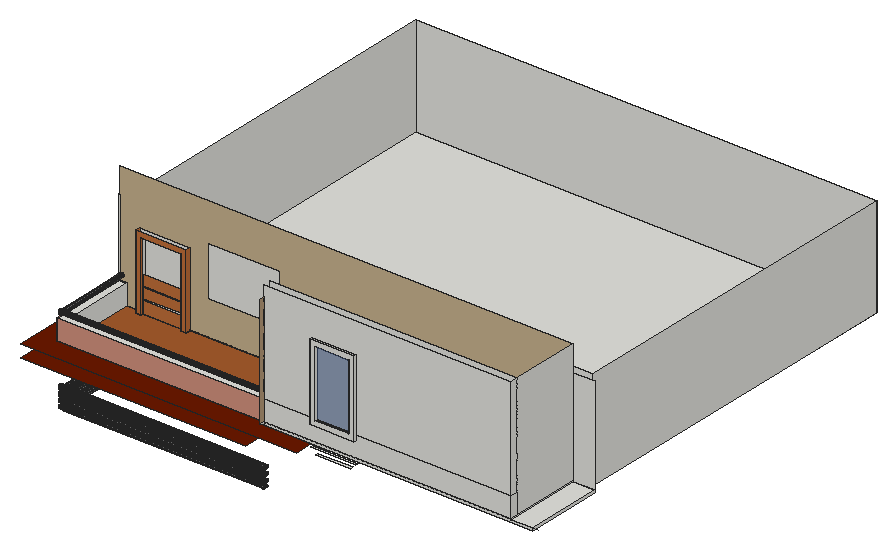
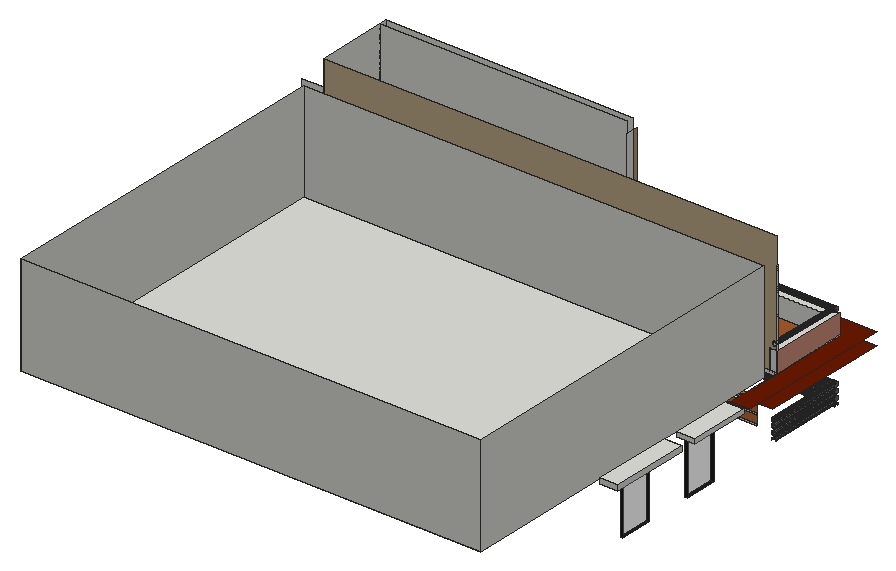
# SketchUp Ruby script. Lengths in inches.
U = 1.inch
M = Sketchup.active_model
def pt(a) = Geom::Point3d.new(a.map { |v| v * U })
def face(e, loops, mat)
  f = e.add_face(loops[0].map { |a| pt(a) })
  loops[1..].each { |l| e.add_face(l.map { |a| pt(a) }).erase! }
  f.material = f.back_material = mat if mat
  f
end
# faces: each face lists its corners as indices into pts; further lists are holes
def faces(e, pts, list, mat = nil) = list.each { |f| face(e, (f[0].is_a?(Array) ? f : [f]).map { |l| l.map { |i| pts[i] } }, mat) }
# xy, xz, yz: faces in a plane at the given z, y or x. An outline is a flat list of corners, or four numbers for a rectangle; further outlines are holes
def ring(l) = l.size == 4 ? [[l[0], l[1]], [l[2], l[1]], [l[2], l[3]], [l[0], l[3]]] : l.each_slice(2).to_a
def flat(e, list, mat, &to3) = list.each { |f| face(e, (f[0].is_a?(Array) ? f : [f]).map { |l| ring(l).map { |u, v| to3.(u, v) } }, mat) }
def xy(e, z, list, mat = nil) = flat(e, list, mat) { |x, y| [x, y, z] }
def xz(e, y, list, mat = nil) = flat(e, list, mat) { |x, z| [x, y, z] }
def yz(e, x, list, mat = nil) = flat(e, list, mat) { |y, z| [x, y, z] }
def lines(e, pts, list) = list.each { |a, b| e.add_line(pt(pts[a]), pt(pts[b])) }
# prism: a flat outline (further loops are holes) pulled along v
def prism(e, loops, v, mat = nil)
  f = face(e, loops, mat); d = Geom::Vector3d.new(v.map { |x| x * U })
  f.pushpull(f.normal.samedirection?(d) ? d.length : -d.length)
end
def box(e, o, s, mat = nil) = prism(e, [[o, [o[0] + s[0], o[1], o[2]], [o[0] + s[0], o[1] + s[1], o[2]], [o[0], o[1] + s[1], o[2]]]], [0, 0, s[2]], mat)
def at(x, y, z, deg = 0) = Geom::Transformation.translation(pt([x, y, z])) * Geom::Transformation.rotation(ORIGIN, Z_AXIS, deg.degrees)
def axes(o, x, y, z) = Geom::Transformation.new([*x, 0, *y, 0, *z, 0, *pt(o).to_a, 1])
def part(name) = M.definitions.add(name)
# library, detail: a bought-in or finely detailed component or shape, given as its bounding box
def library(name, o, s) = part(name).tap { |d| box(d.entities, o, s) }
def detail(e, o, s) = box(e.add_group.entities, o, s)
def put(e, d, t, mat = nil) = e.add_instance(d, t).tap { |i| i.material = mat if mat }
def group(e, t, mat = nil) = e.add_group.tap { |g| g.transformation = t; g.material = mat if mat }.entities
root = M.entities
M.materials.add("[0032_Moccasin]").color = [198, 177, 141]
M.materials.add("[0035_Tan]").color = [181, 154, 120]
M.materials.add("[0134_DimGray]").color = [105, 105, 105]
M.materials.add("[Color B02]").color = [209, 145, 125]
M.materials.add("[Color B07]").color = [107, 26, 0]
M.materials.add("[Color M08]").color = [30, 30, 30]
M.materials.add("[Translucent Glass Blue]").color = [61, 91, 145]
M.materials["[Translucent Glass Blue]"].alpha = 0.5
M.materials.add("[Translucent Glass Gray]").color = [128, 128, 128]
M.materials["[Translucent Glass Gray]"].alpha = 0.5
M.materials.add("[Wood Square Tile 01]").color = [164, 91, 44]
M.materials.add("[Wood Veneer 01]").color = [191, 111, 58]
xy(root,664.14,[[31.875,219.17,34.875,258.48],[31.875,315.92,34.875,355.23]],"[Color M08]")
xy(root,693,[[62.21,116.9375,104.21,119.9375]])
xy(root,693,[[62.21,113.9375,104.21,116.9375]],"[Wood Veneer 01]")
xy(root,699,[[56.21,113.9375,110.21,119.9375]],"[Wood Veneer 01]")
xy(root,706.375,[[144.33,116.9375,184.18,119.9375],[187.18,116.9375,224.02,119.9375]],"[Color M08]")
xy(root,709.375,[[141.33,116.9375,227.02,119.9375]],"[Color M08]")
xy(root,721.21,[[12.5625,0,12.5625,154.8125,34.875,154.8125,34.875,26.9375,282.125,26.9375,282.125,0]],"[Color B07]")
xy(root,727.75,[[31.875,219.17,34.875,258.48],[31.875,315.92,34.875,355.23]],"[Color M08]")
xy(root,728.71,[[352.1,17.9375,393.78,20.9375]])
xy(root,732,[[34.875,26.9375,34.875,119.9375,604.125,119.9375,604.125,35.9375,282.125,35.9375,282.125,26.9375],[282.125,26.9375,604.125,35.9375],[43.875,128.9375,595.125,552.98]])
xy(root,733.75,[[13.875,197.03,13.875,270.28,34.875,270.28,34.875,264.48,31.875,264.48,31.875,213.17,34.875,213.17,34.875,197.03],[31.875,213.17,34.875,264.48],[31.875,309.92,34.875,361.23]])
xy(root,733.87,[[13.875,288.9,34.875,385.9]])
xy(root,734.71,[[346.1,17.9375,399.78,20.9375]])
xy(root,735,[[578.6875,26.9375,604.125,119.9375],[59.96,113.9375,65.96,119.9375],[113.96,113.9375,119.96,119.9375],[65.96,116.9375,113.96,119.9375]])
xy(root,735.99,[[34.875,26.9375,34.875,119.9375,43.875,119.9375,43.875,35.9375,578.6875,35.9375,578.6875,26.9375]])
xy(root,735.99,[[12.5625,0,343.5,0,343.5,20.9375,282.125,20.9375,282.125,26.9375,34.875,26.9375,34.875,189.6875,12.5625,189.6875]],"[Color B07]")
xy(root,735.99,[[43.875,35.9375,578.6875,35.9375,578.6875,119.9375,119.96,119.9375,119.96,113.9375,113.96,113.9375,113.96,116.9375,65.96,116.9375,65.96,113.9375,59.96,113.9375,59.96,119.9375,43.875,119.9375]],"[Wood Square Tile 01]")
xy(root,739.24,[[13.875,197.03,34.875,270.28]])
xy(root,740.24,[[13.875,288.9,34.875,385.9]])
xy(root,758.875,[[344.38,17.9375,398.07,20.9375]])
xy(root,759.99,[[34.875,26.9375,282.125,26.9375,282.125,35.9375,43.875,35.9375,43.875,119.9375,34.875,119.9375],[282.125,26.9375,578.6875,35.9375]])
xy(root,764.875,[[350.38,17.9375,392.07,20.9375]])
xz(root,17.9375,[[[344.38,758.875,398.07,850.6875],[350.38,764.875,392.07,844.6875]]])
xz(root,20.9375,[[[344.38,758.875,398.07,850.6875],[350.38,764.875,392.07,844.6875]]])
xz(root,20.9375,[[350.38,764.875,392.07,844.6875]],"[Translucent Glass Blue]")
xz(root,26.9375,[[34.875,732,282.125,735.99],[282.125,732,282.125,735.99,578.6875,735.99,578.6875,735,604.125,735,604.125,732],[282.125,735.99,578.6875,759.99],[282.125,759.99,578.6875,882.89]])
xz(root,26.9375,[[34.875,735.99,282.125,759.99]],"[Color B02]")
xz(root,26.9375,[[34.875,721.21,282.125,732]],"[Color B07]")
xz(root,30.27,[[38.55,763.37,39.17,763.45,39.74,763.6875,37.36,763.6875,37.9375,763.45],[37.36,763.6875,39.74,763.6875,40.23,764.0625,40.61,764.56,40.85,765.13,40.88,765.43,36.22,765.43,36.26,765.13,36.49,764.56,36.87,764.0625],[36.22,765.43,40.88,765.43,40.93,765.74,40.85,766.36,40.61,766.93,40.23,767.42,39.74,767.8,37.36,767.8,36.87,767.42,36.49,766.93,36.26,766.36,36.18,765.74],[37.36,767.8,39.74,767.8,39.17,768.04,38.55,768.12,37.9375,768.04]])
xz(root,35.9375,[[43.875,735.99,282.125,759.99],[282.125,735.99,578.6875,759.99],[282.125,759.99,578.6875,882.89]])
xz(root,113.9375,[[59.96,735,65.96,735.99],[113.96,735,119.96,735.99]])
xz(root,113.9375,[[59.96,735.99,65.96,735.99,65.96,819,113.96,819,113.96,735.99,119.96,735.99,119.96,825,59.96,825]],"[Wood Veneer 01]")
xz(root,116.9375,[[62.21,668.9375,104.21,670.75],[62.21,681.0625,104.21,682.88],[65.96,735,113.96,735.99],[65.96,751.17,113.96,752.49],[65.96,764.86,113.96,766.18]])
xz(root,116.9375,[[62.21,670.75,104.21,681.0625],[62.21,682.88,104.21,693],[65.96,735.99,113.96,751.17],[65.96,752.49,113.96,764.86],[65.96,766.18,113.96,778.55]],"[Wood Veneer 01]")
xz(root,119.9375,[[59.96,729,119.96,732],[34.875,732,35.6,735.99],[35.6,732,59.96,735.99],[59.96,732,119.96,735],[119.96,732,604.125,732,604.125,735,578.6875,735,578.6875,735.99,119.96,735.99],
  [59.96,735,59.96,825,119.96,825,119.96,735,113.96,735,113.96,819,65.96,819,65.96,735],[65.96,735,113.96,819],[578.6875,735,604.125,852],[34.875,735.99,35.6,759.99],[35.6,735.99,43.875,759.99],
  [34.875,759.99,35.6,852],[38.23,764.56,37.62,764.64,37.04,764.88,36.55,765.26,36.18,765.75,35.9375,766.32,35.86,766.94,35.9375,767.55,36.18,768.12,36.55,768.61,37.04,768.99,37.62,769.23,38.23,769.31,38.85,769.23,39.42,768.99,39.91,768.61,40.29,768.12,40.53,767.55,40.61,766.94,40.53,766.32,40.29,765.75,39.91,765.26,39.42,764.88,38.85,764.64]])
xz(root,119.9375,[[[43.875,735.99,59.96,735.99,59.96,825,119.96,825,119.96,735.99,578.6875,735.99,578.6875,882.89,35.6,882.89,35.6,759.99,43.875,759.99],[141.33,777.125,227.02,837.8125],[38.23,764.56,37.62,764.64,37.04,764.88,36.55,765.26,36.18,765.75,35.9375,766.32,35.86,766.94,35.9375,767.55,36.18,768.12,36.55,768.61,37.04,768.99,37.62,769.23,38.23,769.31,38.85,769.23,39.42,768.99,39.91,768.61,40.29,768.12,40.53,767.55,40.61,766.94,40.53,766.32,40.29,765.75,39.91,765.26,39.42,764.88,38.85,764.64]]],"[0032_Moccasin]")
xz(root,128.9375,[[43.875,732,595.125,852]])
xz(root,197.03,[[13.875,733.75,34.875,739.24]])
xz(root,219.17,[[31.875,664.14,34.875,727.75]],"[Color M08]")
xz(root,258.48,[[31.875,664.14,34.875,727.75]],"[Color M08]")
xz(root,270.28,[[13.875,733.75,34.875,739.24]])
xz(root,288.9,[[13.875,733.87,34.875,740.24]])
xz(root,315.92,[[31.875,664.14,34.875,727.75]],"[Color M08]")
xz(root,355.23,[[31.875,664.14,34.875,727.75]],"[Color M08]")
xz(root,385.9,[[13.875,733.87,34.875,740.24]])
xz(root,552.98,[[43.875,732,595.125,852]])
yz(root,13.875,[[197.03,733.75,270.28,739.24],[288.9,733.87,385.9,740.24]])
yz(root,34.875,[[119.9375,721.21,154.8125,735.99],[26.9375,732,119.9375,735.99]])
yz(root,34.875,[[31.46,667.99,30.85,668.07,30.27,668.3125,29.78,668.6875,29.4,669.18,29.17,669.75,29.09,670.37,29.17,670.98,29.4,671.56,29.78,672.05,30.27,672.42,30.85,672.66,31.46,672.74,32.08,672.66,32.65,672.42,33.14,672.05,33.52,671.56,33.76,670.98,33.84,670.37,33.76,669.75,33.52,669.18,33.14,668.6875,32.65,668.3125,32.08,668.07],[31.46,675.37,30.85,675.45,30.27,675.6875,29.78,676.0625,29.4,676.56,29.17,677.13,29.09,677.74,29.17,678.36,29.4,678.93,29.78,679.42,30.27,679.8,30.85,680.04,31.46,680.12,32.08,680.04,32.65,679.8,33.14,679.42,33.52,678.93,33.76,678.36,33.84,677.74,33.76,677.13,33.52,676.56,33.14,676.0625,32.65,675.6875,32.08,675.45],[31.46,682.74,30.85,682.82,30.27,683.0625,29.78,683.4375,29.4,683.93,29.17,684.5,29.09,685.12,29.17,685.73,29.4,686.31,29.78,686.8,30.27,687.17,30.85,687.41,31.46,687.49,32.08,687.41,32.65,687.17,33.14,686.8,33.52,686.31,33.76,685.73,33.84,685.12,33.76,684.5,33.52,683.93,33.14,683.4375,32.65,683.0625,32.08,682.82],[31.46,763.37,30.85,763.45,30.27,763.6875,29.78,764.0625,29.4,764.56,29.17,765.13,29.09,765.74,29.17,766.36,29.4,766.93,29.78,767.42,30.27,767.8,30.85,768.04,31.46,768.12,32.08,768.04,32.65,767.8,33.14,767.42,33.52,766.93,33.76,766.36,33.84,765.74,33.76,765.13,33.52,764.56,33.14,764.0625,32.65,763.6875,32.08,763.45]],"[0134_DimGray]")
yz(root,34.875,[[26.9375,735.99,119.9375,759.99]],"[Color B02]")
yz(root,34.875,[[26.9375,721.21,119.9375,732]],"[Color B07]")
yz(root,34.875,[[219.17,664.14,258.48,727.75],[315.92,664.14,355.23,727.75]],"[Translucent Glass Gray]")
yz(root,43.875,[[128.9375,732,552.98,852],[35.9375,735.99,119.9375,759.99]])
yz(root,59.96,[[113.9375,735,119.9375,735.99]])
yz(root,59.96,[[113.9375,735.99,119.9375,825]],"[Wood Veneer 01]")
yz(root,65.96,[[113.9375,735,116.9375,735.99],[116.9375,735,119.9375,819]])
yz(root,65.96,[[113.9375,735.99,116.9375,819]],"[Wood Veneer 01]")
yz(root,113.96,[[113.9375,735,116.9375,735.99],[116.9375,735,119.9375,819]])
yz(root,113.96,[[113.9375,735.99,116.9375,819]],"[Wood Veneer 01]")
yz(root,119.96,[[113.9375,735,119.9375,735.99]])
yz(root,119.96,[[113.9375,735.99,119.9375,825]],"[Wood Veneer 01]")
yz(root,282.125,[[20.9375,721.21,26.9375,735.99],[26.9375,721.21,35.9375,732],[[26.9375,759.99,35.9375,869.45],[31.46,770.43,32.08,770.51,32.65,770.75,33.14,771.125,33.52,771.62,33.76,772.19,33.84,772.81,33.76,773.42,33.52,773.99,33.14,774.48,32.65,774.86,32.08,775.1,31.46,775.18,30.85,775.1,30.27,774.86,29.78,774.48,29.4,773.99,29.17,773.42,29.09,772.81,29.17,772.19,29.4,771.62,29.78,771.125,30.27,770.75,30.85,770.51],[31.46,777.49,32.08,777.57,32.65,777.8125,33.14,778.1875,33.52,778.68,33.76,779.25,33.84,779.87,33.76,780.48,33.52,781.06,33.14,781.55,32.65,781.92,32.08,782.16,31.46,782.24,30.85,782.16,30.27,781.92,29.78,781.55,29.4,781.06,29.17,780.48,29.09,779.87,29.17,779.25,29.4,778.68,29.78,778.1875,30.27,777.8125,30.85,777.57],[31.46,784.56,32.08,784.64,32.65,784.875,33.14,785.25,33.52,785.74,33.76,786.32,33.84,786.93,33.76,787.54,33.52,788.12,33.14,788.61,32.65,788.99,32.08,789.22,31.46,789.31,30.85,789.22,30.27,788.99,29.78,788.61,29.4,788.12,29.17,787.54,29.09,786.93,29.17,786.32,29.4,785.74,29.78,785.25,30.27,784.875,30.85,784.64],[31.46,791.62,32.08,791.7,32.65,791.9375,33.14,792.3125,33.52,792.81,33.76,793.38,33.84,793.99,33.76,794.61,33.52,795.18,33.14,795.67,32.65,796.05,32.08,796.29,31.46,796.37,30.85,796.29,30.27,796.05,29.78,795.67,29.4,795.18,29.17,794.61,29.09,793.99,29.17,793.38,29.4,792.81,29.78,792.3125,30.27,791.9375,30.85,791.7],[31.46,763.37,32.08,763.45,32.65,763.6875,33.14,764.0625,33.52,764.56,33.76,765.13,33.84,765.74,33.76,766.36,33.52,766.93,33.14,767.42,32.65,767.8,32.08,768.04,31.46,768.12,30.85,768.04,30.27,767.8,29.78,767.42,29.4,766.93,29.17,766.36,29.09,765.74,29.17,765.13,29.4,764.56,29.78,764.0625,30.27,763.6875,30.85,763.45]],[31.46,763.37,32.08,763.45,32.65,763.6875,33.14,764.0625,33.52,764.56,33.76,765.13,33.84,765.74,33.76,766.36,33.52,766.93,33.14,767.42,32.65,767.8,32.08,768.04,31.46,768.12,30.85,768.04,30.27,767.8,29.78,767.42,29.4,766.93,29.17,766.36,29.09,765.74,29.17,765.13,29.4,764.56,29.78,764.0625,30.27,763.6875,30.85,763.45]])
yz(root,282.125,[[20.9375,735.99,26.9375,869.45]],"[0035_Tan]")
yz(root,344.38,[[17.9375,758.875,20.9375,850.6875]])
yz(root,350.38,[[17.9375,764.875,20.9375,844.6875]])
yz(root,392.07,[[17.9375,764.875,20.9375,844.6875]])
yz(root,398.07,[[17.9375,758.875,20.9375,850.6875]])
yz(root,578.6875,[[26.9375,735,119.9375,735.99],[26.9375,735.99,35.9375,759.99],[35.9375,735.99,119.9375,882.89],[26.9375,759.99,35.9375,882.89]])
yz(root,595.125,[[128.9375,732,552.98,852]])
yz(root,604.125,[[26.9375,732,119.9375,735]])
p = [[282.125,29.17,662.38],[282.125,29.09,662.99],[34.875,29.09,662.99],[34.875,29.17,662.38],[37.3,29.17,662.38],[41.84,29.17,662.38],
  [37.19,119.9375,663.05],[37.27,119.9375,662.4375],[37.27,29.17,662.4375],[37.19,29.17,663.05],[41.86,119.9375,662.4375],[41.94,119.9375,663.05],
  [41.94,29.17,663.05],[41.86,29.17,662.4375],[282.125,33.84,662.99],[282.125,33.76,662.38],[34.875,33.76,662.38],[34.875,33.84,662.99],
  [282.125,29.17,663.61],[41.87,29.17,663.61],[37.27,29.17,663.61],[34.875,29.17,663.61],[282.125,33.76,663.61],[34.875,33.76,663.61],
  [37.27,119.9375,663.67],[37.24,29.17,663.42],[37.27,29.17,663.67],[41.86,119.9375,663.67],[41.86,29.17,663.67],[41.89,29.17,663.42],
  [282.125,29.4,664.18],[34.875,29.4,664.18],[282.125,33.52,664.18],[34.875,33.52,664.18],[37.51,119.9375,664.24],[37.51,29.17,664.24],
  [41.625,119.9375,664.24],[41.625,29.17,664.24],[37.89,119.9375,664.73],[37.89,29.17,664.73],[41.25,119.9375,664.73],[41.25,29.17,664.73],
  [282.125,29.78,664.67],[34.875,29.78,664.67],[282.125,33.14,664.67],[34.875,33.14,664.67],[38.38,119.9375,665.11],[38.38,29.17,665.11],
  [40.76,119.9375,665.11],[40.76,29.17,665.11],[282.125,30.27,665.05],[34.875,30.27,665.05],[282.125,32.65,665.05],[34.875,32.65,665.05],
  [282.125,30.85,665.29],[34.875,30.85,665.29],[282.125,32.08,665.29],[34.875,32.08,665.29],[38.95,119.9375,665.35],[38.95,29.17,665.35],
  [40.18,119.9375,665.35],[40.18,29.17,665.35],[39.57,119.9375,665.43],[39.57,29.17,665.43],[282.125,31.46,665.37],[34.875,31.46,665.37],
  [282.125,31.46,667.99],[282.125,30.85,668.07],[34.875,30.85,668.07],[34.875,31.46,667.99],[282.125,32.08,668.07],[34.875,32.08,668.07],
  [38.95,119.9375,668.2],[39.57,119.9375,668.12],[39.57,29.17,668.12],[38.95,29.17,668.2],[40.18,119.9375,668.2],[40.18,29.17,668.2],
  [282.125,30.27,668.3125],[34.875,30.27,668.3125],[282.125,32.65,668.3125],[34.875,32.65,668.3125],[38.38,119.9375,668.43],[38.38,29.17,668.43],
  [40.76,119.9375,668.43],[40.76,29.17,668.43],[282.125,29.78,668.6875],[34.875,29.78,668.6875],[282.125,33.14,668.6875],[34.875,33.14,668.6875],
  [37.89,119.9375,668.8125],[37.89,29.17,668.8125],[41.25,119.9375,668.8125],[41.25,29.17,668.8125],[282.125,29.4,669.18],[34.875,29.4,669.18],
  [282.125,33.52,669.18],[34.875,33.52,669.18],[37.51,119.9375,669.3],[37.51,29.17,669.3],[41.625,119.9375,669.3],[41.625,29.17,669.3],
  [282.125,29.17,669.75],[41.8125,29.17,669.75],[37.32,29.17,669.75],[34.875,29.17,669.75],[282.125,33.76,669.75],[34.875,33.76,669.75],
  [37.27,119.9375,669.875],[37.375,29.17,669.63],[37.3,29.17,669.82],[37.27,29.17,669.875],[41.86,119.9375,669.875],[41.86,29.17,669.875],
  [41.84,29.17,669.82],[41.76,29.17,669.63],[282.125,29.09,670.37],[34.875,29.09,670.37],[282.125,33.84,670.37],[34.875,33.84,670.37],
  [37.19,119.9375,670.49],[37.19,29.17,670.49],[41.94,119.9375,670.49],[41.94,29.17,670.49],[282.125,29.17,670.98],[41.88,29.17,670.98],
  [37.26,29.17,670.98],[34.875,29.17,670.98],[282.125,33.76,670.98],[34.875,33.76,670.98],[37.27,119.9375,671.11],[37.24,29.17,670.86],
  [37.27,29.17,671.04],[37.27,29.17,671.11],[41.86,119.9375,671.11],[41.86,29.17,671.11],[41.87,29.17,671.04],[41.89,29.17,670.86],
  [282.125,29.4,671.56],[34.875,29.4,671.56],[282.125,33.52,671.56],[34.875,33.52,671.56],[37.51,119.9375,671.68],[37.51,29.17,671.68],
  [41.625,119.9375,671.68],[41.625,29.17,671.68],[282.125,29.78,672.05],[34.875,29.78,672.05],[282.125,33.14,672.05],[34.875,33.14,672.05],
  [37.89,119.9375,672.17],[37.89,29.17,672.17],[41.25,119.9375,672.17],[41.25,29.17,672.17],[282.125,30.27,672.42],[34.875,30.27,672.42],
  [282.125,32.65,672.42],[34.875,32.65,672.42],[38.38,119.9375,672.55],[38.38,29.17,672.55],[40.76,119.9375,672.55],[40.76,29.17,672.55],
  [282.125,30.85,672.66],[34.875,30.85,672.66],[282.125,32.08,672.66],[34.875,32.08,672.66],[38.95,119.9375,672.79],[38.95,29.17,672.79],
  [40.18,119.9375,672.79],[40.18,29.17,672.79],[282.125,31.46,672.74],[34.875,31.46,672.74],[39.57,119.9375,672.87],[39.57,29.17,672.87],
  [282.125,30.85,675.45],[282.125,30.27,675.6875],[34.875,30.27,675.6875],[34.875,30.85,675.45],[282.125,31.46,675.37],[34.875,31.46,675.37],
  [282.125,32.08,675.45],[34.875,32.08,675.45],[282.125,32.65,675.6875],[34.875,32.65,675.6875],[38.38,119.9375,675.87],[38.95,119.9375,675.63],
  [38.95,29.17,675.63],[38.38,29.17,675.87],[39.57,119.9375,675.55],[39.57,29.17,675.55],[40.18,119.9375,675.63],[40.18,29.17,675.63],
  [40.76,119.9375,675.87],[40.76,29.17,675.87],[282.125,29.78,676.0625],[34.875,29.78,676.0625],[282.125,33.14,676.0625],[34.875,33.14,676.0625],
  [37.89,119.9375,676.25],[37.89,29.17,676.25],[41.25,119.9375,676.25],[41.25,29.17,676.25],[282.125,29.4,676.56],[34.875,29.4,676.56],
  [282.125,33.52,676.56],[34.875,33.52,676.56],[37.51,119.9375,676.74],[37.51,29.17,676.74],[41.625,119.9375,676.74],[41.625,29.17,676.74],
  [282.125,29.17,677.13],[41.78,29.17,677.13],[37.35,29.17,677.13],[34.875,29.17,677.13],[282.125,33.76,677.13],[34.875,33.76,677.13],
  [37.27,119.9375,677.3125],[37.375,29.17,677.07],[37.32,29.17,677.19],[37.3,29.17,677.25],[37.27,29.17,677.3125],[41.86,119.9375,677.3125],
  [41.86,29.17,677.3125],[41.84,29.17,677.25],[41.8125,29.17,677.19],[41.76,29.17,677.07],[282.125,29.09,677.74],[34.875,29.09,677.74],
  [282.125,33.84,677.74],[34.875,33.84,677.74],[37.19,119.9375,677.93],[37.19,29.17,677.93],[41.94,119.9375,677.93],[41.94,29.17,677.93],
  [282.125,29.17,678.36],[41.89,29.17,678.36],[37.25,29.17,678.36],[34.875,29.17,678.36],[282.125,33.76,678.36],[34.875,33.76,678.36],
  [37.27,119.9375,678.54],[37.24,29.17,678.29],[37.26,29.17,678.42],[37.27,29.17,678.48],[37.27,29.17,678.54],[41.86,119.9375,678.54],
  [41.86,29.17,678.54],[41.87,29.17,678.48],[41.88,29.17,678.42],[41.89,29.17,678.29],[282.125,29.4,678.93],[34.875,29.4,678.93],
  [282.125,33.52,678.93],[34.875,33.52,678.93],[37.51,119.9375,679.12],[37.51,29.17,679.12],[41.625,119.9375,679.12],[41.625,29.17,679.12],
  [282.125,29.78,679.42],[34.875,29.78,679.42],[282.125,33.14,679.42],[34.875,33.14,679.42],[37.89,119.9375,679.61],[37.89,29.17,679.61],
  [41.25,119.9375,679.61],[41.25,29.17,679.61],[282.125,30.27,679.8],[34.875,30.27,679.8],[282.125,32.65,679.8],[34.875,32.65,679.8],
  [38.38,119.9375,679.99],[38.38,29.17,679.99],[40.76,119.9375,679.99],[40.76,29.17,679.99],[282.125,30.85,680.04],[34.875,30.85,680.04],
  [282.125,32.08,680.04],[34.875,32.08,680.04],[38.95,119.9375,680.22],[38.95,29.17,680.22],[40.18,119.9375,680.22],[40.18,29.17,680.22],
  [282.125,31.46,680.12],[34.875,31.46,680.12],[39.57,119.9375,680.3],[39.57,29.17,680.3],[38.95,119.9375,682.57],[39.57,119.9375,682.49],
  [39.57,29.17,682.49],[38.95,29.17,682.57],[40.18,119.9375,682.57],[40.18,29.17,682.57],[38.38,119.9375,682.81],[38.38,29.17,682.81],
  [40.76,119.9375,682.81],[40.76,29.17,682.81],[282.125,31.46,682.74],[282.125,30.85,682.82],[34.875,30.85,682.82],[34.875,31.46,682.74],
  [282.125,32.08,682.82],[34.875,32.08,682.82],[37.89,119.9375,683.1875],[37.89,29.17,683.1875],[41.25,119.9375,683.1875],[41.25,29.17,683.1875],
  [282.125,30.27,683.0625],[34.875,30.27,683.0625],[282.125,32.65,683.0625],[34.875,32.65,683.0625],[282.125,29.78,683.4375],[34.875,29.78,683.4375],
  [282.125,33.14,683.4375],[34.875,33.14,683.4375],[37.51,119.9375,683.68],[37.51,29.17,683.68],[41.625,119.9375,683.68],[41.625,29.17,683.68],
  [282.125,29.4,683.93],[34.875,29.4,683.93],[282.125,33.52,683.93],[34.875,33.52,683.93],[37.27,119.9375,684.25],[37.375,29.17,684],
  [37.35,29.17,684.07],[37.32,29.17,684.13],[37.3,29.17,684.19],[37.27,29.17,684.25],[41.86,119.9375,684.25],[41.86,29.17,684.25],
  [41.84,29.17,684.19],[41.8125,29.17,684.13],[41.78,29.17,684.07],[41.76,29.17,684],[282.125,29.17,684.5],[41.9,29.17,684.5],
  [37.24,29.17,684.5],[34.875,29.17,684.5],[282.125,33.76,684.5],[34.875,33.76,684.5],[37.19,119.9375,684.87],[37.19,29.17,684.87],
  [41.94,119.9375,684.87],[41.94,29.17,684.87],[282.125,29.09,685.12],[34.875,29.09,685.12],[282.125,33.84,685.12],[34.875,33.84,685.12],
  [37.27,119.9375,685.48],[37.24,29.17,685.23],[37.25,29.17,685.29],[37.26,29.17,685.36],[37.27,29.17,685.42],[37.27,29.17,685.48],
  [41.86,119.9375,685.48],[41.86,29.17,685.48],[41.87,29.17,685.42],[41.88,29.17,685.36],[41.89,29.17,685.29],[41.89,29.17,685.23],
  [282.125,29.17,685.73],[41.76,29.17,685.73],[37.38,29.17,685.73],[34.875,29.17,685.73],[282.125,33.76,685.73],[34.875,33.76,685.73],
  [37.51,119.9375,686.05],[37.51,29.17,686.05],[41.625,119.9375,686.05],[41.625,29.17,686.05],[282.125,29.4,686.31],[34.875,29.4,686.31],
  [282.125,33.52,686.31],[34.875,33.52,686.31],[37.89,119.9375,686.55],[37.89,29.17,686.55],[41.25,119.9375,686.55],[41.25,29.17,686.55],
  [282.125,29.78,686.8],[34.875,29.78,686.8],[282.125,33.14,686.8],[34.875,33.14,686.8],[38.38,119.9375,686.92],[38.38,29.17,686.92],
  [40.76,119.9375,686.92],[40.76,29.17,686.92],[282.125,30.27,687.17],[34.875,30.27,687.17],[282.125,32.65,687.17],[34.875,32.65,687.17],
  [38.95,119.9375,687.16],[38.95,29.17,687.16],[40.18,119.9375,687.16],[40.18,29.17,687.16],[39.57,119.9375,687.24],[39.57,29.17,687.24],
  [282.125,30.85,687.41],[34.875,30.85,687.41],[282.125,32.08,687.41],[34.875,32.08,687.41],[282.125,31.46,687.49],[34.875,31.46,687.49],
  [36.22,30.27,765.43],[34.875,31.46,763.37],[282.125,32.08,763.45],[34.875,30.85,763.45],[282.125,30.85,763.45],[282.125,30.27,763.6875],
  [39.74,30.27,763.6875],[37.36,30.27,763.6875],[34.875,30.27,763.6875],[40.88,30.27,765.43],[37.04,119.9375,764.88],[37.62,119.9375,764.64],
  [37.9375,30.27,763.45],[38.23,119.9375,764.56],[38.55,30.27,763.37],[38.85,119.9375,764.64],[39.17,30.27,763.45],[39.42,119.9375,764.88],
  [282.125,31.46,763.37],[34.875,32.08,763.45],[282.125,32.65,763.6875],[34.875,32.65,763.6875],[282.125,29.78,764.0625],[34.875,29.78,764.0625],
  [36.55,119.9375,765.26],[36.87,30.27,764.0625],[39.91,119.9375,765.26],[40.23,30.27,764.0625],[282.125,33.14,764.0625],[34.875,33.14,764.0625],
  [282.125,29.4,764.56],[34.875,29.4,764.56],[36.49,30.27,764.56],[36.18,119.9375,765.75],[40.29,119.9375,765.75],[40.61,30.27,764.56],
  [282.125,33.52,764.56],[34.875,33.52,764.56],[282.125,29.17,765.13],[34.875,29.17,765.13],[36.26,30.27,765.13],[35.9375,119.9375,766.32],
  [40.53,119.9375,766.32],[40.85,30.27,765.13],[282.125,33.76,765.13],[34.875,33.76,765.13],[282.125,29.09,765.74],[34.875,29.09,765.74],
  [36.18,30.27,765.74],[35.86,119.9375,766.94],[40.61,119.9375,766.94],[40.93,30.27,765.74],[282.125,33.84,765.74],[34.875,33.84,765.74],
  [282.125,29.17,766.36],[34.875,29.17,766.36],[36.26,30.27,766.36],[35.9375,119.9375,767.55],[40.53,119.9375,767.55],[40.85,30.27,766.36],
  [282.125,33.76,766.36],[34.875,33.76,766.36],[282.125,29.4,766.93],[34.875,29.4,766.93],[36.49,30.27,766.93],[36.18,119.9375,768.12],
  [40.29,119.9375,768.12],[40.61,30.27,766.93],[282.125,33.52,766.93],[34.875,33.52,766.93],[282.125,29.78,767.42],[34.875,29.78,767.42],
  [36.87,30.27,767.42],[36.55,119.9375,768.61],[39.91,119.9375,768.61],[40.23,30.27,767.42],[282.125,33.14,767.42],[34.875,33.14,767.42],
  [282.125,30.27,767.8],[39.74,30.27,767.8],[37.36,30.27,767.8],[34.875,30.27,767.8],[37.04,119.9375,768.99],[39.42,119.9375,768.99],
  [282.125,32.65,767.8],[34.875,32.65,767.8],[282.125,30.85,768.04],[34.875,30.85,768.04],[37.9375,30.27,768.04],[37.62,119.9375,769.23],
  [38.85,119.9375,769.23],[39.17,30.27,768.04],[282.125,32.08,768.04],[34.875,32.08,768.04],[38.55,30.27,768.12],[38.23,119.9375,769.31],
  [282.125,31.46,768.12],[34.875,31.46,768.12],[604.125,26.9375,735],[610.875,26.9375,735]]
faces(root,p,[[0,1,2,3,4,5],[6,7,8,9],[10,11,12,13],[14,15,16,17],[1,18,19,20,21,2],[22,14,17,23],[24,6,9,25,20,26],[11,27,28,19,29,12],
  [18,30,31,21,20,19],[32,22,23,33],[34,24,26,35],[27,36,37,28],[38,34,35,39],[36,40,41,37],[30,42,43,31],[44,32,33,45],
  [46,38,39,47],[40,48,49,41],[42,50,51,43],[52,44,45,53],[50,54,55,51],[56,52,53,57],[58,46,47,59],[48,60,61,49],
  [62,58,59,63],[60,62,63,61],[54,64,65,55],[64,56,57,65],[66,67,68,69],[70,66,69,71],[72,73,74,75],[73,76,77,74],
  [67,78,79,68],[80,70,71,81],[82,72,75,83],[76,84,85,77],[78,86,87,79],[88,80,81,89],[90,82,83,91],[84,92,93,85],
  [86,94,95,87],[96,88,89,97],[98,90,91,99],[92,100,101,93],[94,102,103,104,105,95],[106,96,97,107],[108,98,99,109,104,110,111],[100,112,113,114,103,115,101],
  [102,116,117,105,104,103],[118,106,107,119],[120,108,111,121],[112,122,123,113],[116,124,125,126,127,117],[128,118,119,129],[130,120,121,131,126,132,133],[122,134,135,136,125,137,123],
  [124,138,139,127,126,125],[140,128,129,141],[142,130,133,143],[134,144,145,135],[138,146,147,139],[148,140,141,149],[150,142,143,151],[144,152,153,145],
  [146,154,155,147],[156,148,149,157],[158,150,151,159],[152,160,161,153],[154,162,163,155],[164,156,157,165],[166,158,159,167],[160,168,169,161],
  [162,170,171,163],[170,164,165,171],[172,166,167,173],[168,172,173,169],[174,175,176,177],[178,174,177,179],[180,178,179,181],[182,180,181,183],
  [184,185,186,187],[185,188,189,186],[188,190,191,189],[190,192,193,191],[175,194,195,176],[196,182,183,197],[198,184,187,199],[192,200,201,193],
  [194,202,203,195],[204,196,197,205],[206,198,199,207],[200,208,209,201],[202,210,211,212,213,203],[214,204,205,215],[216,206,207,217,212,218,219,220],[208,221,222,223,224,211,225,209],
  [210,226,227,213,212,211],[228,214,215,229],[230,216,220,231],[221,232,233,222],[226,234,235,236,237,227],[238,228,229,239],[240,230,231,241,236,242,243,244],[232,245,246,247,248,235,249,233],
  [234,250,251,237,236,235],[252,238,239,253],[254,240,244,255],[245,256,257,246],[250,258,259,251],[260,252,253,261],[262,254,255,263],[256,264,265,257],
  [258,266,267,259],[268,260,261,269],[270,262,263,271],[264,272,273,265],[266,274,275,267],[276,268,269,277],[278,270,271,279],[272,280,281,273],
  [274,282,283,275],[282,276,277,283],[284,278,279,285],[280,284,285,281],[286,287,288,289],[287,290,291,288],[292,286,289,293],[290,294,295,291],
  [296,297,298,299],[300,296,299,301],[302,292,293,303],[294,304,305,295],[297,306,307,298],[308,300,301,309],[306,310,311,307],[312,308,309,313],
  [314,302,303,315],[304,316,317,305],[310,318,319,311],[320,312,313,321],[322,314,315,323,324,325,326,327],[316,328,329,330,331,332,333,317],[318,334,335,336,337,319],[338,320,321,339],
  [340,322,327,336,341],[328,342,343,335,329],[334,344,345,337,336,335],[346,338,339,347],[348,340,341,349,350,351,352,353],[342,354,355,356,357,358,359,343],[344,360,361,362,363,345],[364,346,347,365],
  [366,348,353,362,367],[354,368,369,361,355],[360,370,371,363,362,361],[372,364,365,373],[374,366,367,375],[368,376,377,369],[370,378,379,371],[380,372,373,381],
  [382,374,375,383],[376,384,385,377],[378,386,387,379],[388,380,381,389],[390,382,383,391],[384,392,393,385],[394,390,391,395],[392,394,395,393],
  [386,396,397,387],[398,388,389,399],[396,400,401,397],[400,398,399,401],[402,403,404],[403,402,405],[406,407,408,409,410,405],[405,402,411,406],
  [411,402,404],[412,413,414,409],[413,415,416,414],[415,417,418,416],[417,419,408,418],[420,411,404],[420,406,411],[421,404,403],
  [422,404,421,423],[407,424,425,410,409,408],[426,412,409,427],[419,428,429,408],[430,422,423,431],[424,432,433,425],[434,435,426,427],[429,428,436,437],
  [438,430,431,439],[432,440,441,433],[442,443,435,434],[437,436,444,445],[446,438,439,447],[440,448,449,441],[450,451,443,442,402],[445,444,452,453,411],
  [454,446,447,455],[448,456,457,449],[458,459,451,450],[453,452,460,461],[462,454,455,463],[456,464,465,457],[466,467,459,458],[461,460,468,469],
  [470,462,463,471],[464,472,473,465],[474,475,467,466],[469,468,476,477],[478,470,471,479],[472,480,481,482,483,473],[475,474,482,484],[485,481,477,476],
  [486,478,479,487],[480,488,489,483,482,481],[484,482,490,491],[492,493,481,485],[494,486,487,495],[491,490,496,497],[497,496,493,492],[488,498,499,489],
  [498,494,495,499]],"[0134_DimGray]")
lines(root,p,[[500,501]])
